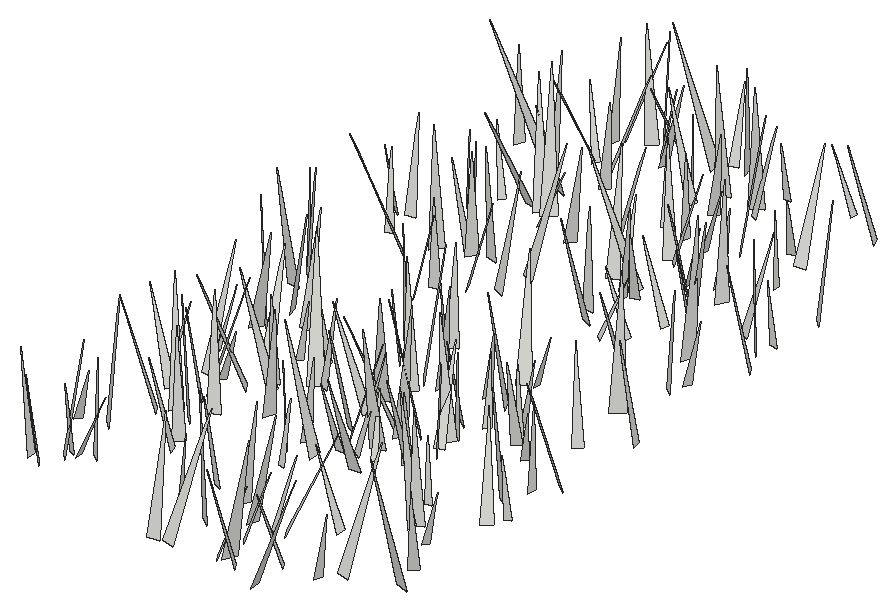
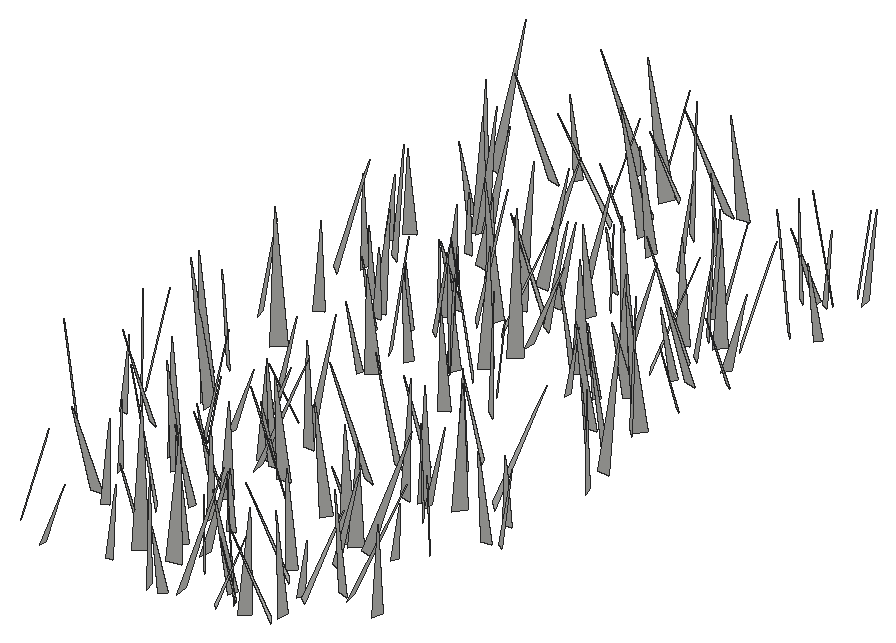
# SketchUp Ruby script. Lengths in inches.
U = 1.inch
M = Sketchup.active_model
def pt(a) = Geom::Point3d.new(a.map { |v| v * U })
def face(e, loops, mat)
  f = e.add_face(loops[0].map { |a| pt(a) })
  loops[1..].each { |l| e.add_face(l.map { |a| pt(a) }).erase! }
  f.material = f.back_material = mat if mat
  f
end
# faces: each face lists its corners as indices into pts; further lists are holes
def faces(e, pts, list, mat = nil) = list.each { |f| face(e, (f[0].is_a?(Array) ? f : [f]).map { |l| l.map { |i| pts[i] } }, mat) }
# xy, xz, yz: faces in a plane at the given z, y or x. An outline is a flat list of corners, or four numbers for a rectangle; further outlines are holes
def ring(l) = l.size == 4 ? [[l[0], l[1]], [l[2], l[1]], [l[2], l[3]], [l[0], l[3]]] : l.each_slice(2).to_a
def flat(e, list, mat, &to3) = list.each { |f| face(e, (f[0].is_a?(Array) ? f : [f]).map { |l| ring(l).map { |u, v| to3.(u, v) } }, mat) }
def xy(e, z, list, mat = nil) = flat(e, list, mat) { |x, y| [x, y, z] }
def xz(e, y, list, mat = nil) = flat(e, list, mat) { |x, z| [x, y, z] }
def yz(e, x, list, mat = nil) = flat(e, list, mat) { |y, z| [x, y, z] }
def lines(e, pts, list) = list.each { |a, b| e.add_line(pt(pts[a]), pt(pts[b])) }
# prism: a flat outline (further loops are holes) pulled along v
def prism(e, loops, v, mat = nil)
  f = face(e, loops, mat); d = Geom::Vector3d.new(v.map { |x| x * U })
  f.pushpull(f.normal.samedirection?(d) ? d.length : -d.length)
end
def box(e, o, s, mat = nil) = prism(e, [[o, [o[0] + s[0], o[1], o[2]], [o[0] + s[0], o[1] + s[1], o[2]], [o[0], o[1] + s[1], o[2]]]], [0, 0, s[2]], mat)
def at(x, y, z, deg = 0) = Geom::Transformation.translation(pt([x, y, z])) * Geom::Transformation.rotation(ORIGIN, Z_AXIS, deg.degrees)
def axes(o, x, y, z) = Geom::Transformation.new([*x, 0, *y, 0, *z, 0, *pt(o).to_a, 1])
def part(name) = M.definitions.add(name)
# library, detail: a bought-in or finely detailed component or shape, given as its bounding box
def library(name, o, s) = part(name).tap { |d| box(d.entities, o, s) }
def detail(e, o, s) = box(e.add_group.entities, o, s)
def put(e, d, t, mat = nil) = e.add_instance(d, t).tap { |i| i.material = mat if mat }
def group(e, t, mat = nil) = e.add_group.tap { |g| g.transformation = t; g.material = mat if mat }.entities
root = M.entities
c1 = part("fur_instance\#9")
p = [[0.8125,0,1.79],[0.67,-0.02,1.48],[0,-0.11,0],[0,0.11,0]]
faces(c1.entities,p,[[0,1,2,3]])
put(root,c1,axes([454.9,228.46,-21.66],[-2.14945,-3.42966,1.0737],[-3.50191,2.27993,0.27214],[0.80747,0.75821,4.03839]))
put(root,c1,axes([455.0625,214.63,-21.66],[-4.85936,-1.80324,2.4582],[-1.94231,5.39639,0.11902],[2.34986,0.73149,5.18178]))
put(root,c1,axes([455.69,246.77,-21.66],[-4.75498,1.70819,1.94206],[1.76287,5.11453,-0.18234],[1.89256,-0.47231,5.04921]))
put(root,c1,axes([456.17,210.82,-21.66],[-0.95753,-7.17721,1.84222],[-7.39469,1.0444,0.22542],[0.47406,1.79439,7.23729]))
put(root,c1,axes([456.03,213.25,-21.66],[3.99026,4.07334,2.14881],[4.32029,-4.29562,0.12027],[-1.59518,-1.44473,5.70086]))
put(root,c1,axes([456.43,228.82,-21.66],[-1.35199,5.16754,1.66066],[5.39955,1.4549,-0.13134],[0.55327,-1.57128,5.33986]))
put(root,c1,axes([457.3,168.51,-21.66],[4.90342,0.51596,3.18153],[0.4361,-5.84514,0.27581],[-3.19346,-0.00597,4.92277]))
put(root,c1,axes([456.92,224.95,-21.66],[-1.17354,4.22506,1.16991],[4.38332,1.15287,0.2334],[0.0799,-1.19029,4.3788]))
put(root,c1,axes([459.98,245.51,-21.66],[-7.66892,-1.90839,0.15613],[-1.91216,7.66661,-0.21311],[0.09999,0.24454,7.89993]))
put(root,c1,axes([456.22,177.14,-21.66],[3.1539,-2.32332,0.00557],[-2.32207,-3.15188,0.13648],[0.07647,0.11319,3.91488]))
put(root,c1,axes([459.46,187.51,-21.66],[-4.99004,2.24313,0.58277],[2.2784,5.00139,0.2583],[0.42444,-0.4756,5.46492]))
put(root,c1,axes([457.4375,189.73,-21.66],[2.29816,3.3477,0.63042],[3.39972,-2.30202,-0.16916],[-0.21536,-0.61617,4.05709]))
put(root,c1,axes([458.8125,167.71,-21.66],[3.31439,2.62679,2.62231],[3.03004,-3.94532,0.12232],[-2.14367,-1.5153,4.22732]))
put(root,c1,axes([460.44,222.64,-21.66],[-5.16383,-5.19186,0.43743],[-5.2089,5.15828,-0.26709],[0.11856,0.49863,7.31773]))
put(root,c1,axes([458.3,196.53,-21.66],[2.21445,2.95218,0.72503],[3.03203,-2.20951,-0.26401],[-0.21871,-0.73996,3.68096]))
put(root,c1,axes([459.07,202.87,-21.66],[-4.9247,-5.05159,2.9073],[-5.39927,5.38751,0.21521],[2.19519,1.91829,7.05159]))
put(root,c1,axes([459.38,233.9,-21.66],[3.09242,2.58599,1.68004],[2.84079,-3.31463,-0.12697],[-1.19992,-1.18273,4.02918]))
put(root,c1,axes([459.37,177.89,-21.66],[4.78863,4.89843,2.46119],[5.13986,-5.14824,0.24599],[-1.90629,-1.57608,6.84581]))
put(root,c1,axes([461.24,183.1,-21.66],[-5.49942,-3.45806,0.94275],[-3.51329,5.5426,-0.16378],[0.70973,0.64178,6.49422]))
put(root,c1,axes([459.34,206.71,-21.66],[5.12051,1.66894,1.66295],[1.70709,-5.37015,0.13306],[-1.62376,-0.38277,5.38398]))
put(root,c1,axes([460.07,171.33,-21.66],[-1.89592,-3.45095,1.30694],[-3.60556,2.04518,0.16982],[0.78554,1.05823,3.9338]))
put(root,c1,axes([461.32,236.99,-21.66],[-3.55756,1.9012,0.49829],[1.88183,3.59228,-0.2708],[0.56709,0.00632,4.02461]))
put(root,c1,axes([458.44,202.23,-21.66],[5.57249,-4.36069,0.56036],[-4.38496,-5.5781,0.19774],[-0.31889,0.50141,7.07313]))
put(root,c1,axes([459.89,170.41,-21.66],[-4.21577,-3.58718,3.5566],[-4.31781,4.96325,-0.11214],[2.62178,2.40587,5.53425]))
put(root,c1,axes([460.59,191.79,-21.66],[0.90222,6.95991,0.72818],[6.98982,-0.93156,0.24337],[-0.33621,-0.69025,7.01392]))
put(root,c1,axes([460.99,245.52,-21.66],[1.59622,5.71911,2.00108],[6.0184,-1.73595,0.16062],[-0.70101,-1.88115,5.93551]))
put(root,c1,axes([462.76,184.31,-21.66],[-5.4488,4.52209,1.619],[4.59694,5.6194,-0.22458],[1.39234,-0.85616,7.07731]))
put(root,c1,axes([463.16,248.99,-21.66],[-3.18461,-4.17271,0.10236],[-4.17132,3.18622,0.10881],[0.1486,0.01532,5.24799]))
put(root,c1,axes([462.46,225.35,-21.66],[-4.98307,4.13485,3.06586],[4.6284,5.46651,0.15019],[2.25263,-2.08511,6.47344]))
put(root,c1,axes([460.98,171.3,-21.66],[4.07736,0.20577,0.16386],[0.20057,-4.0788,0.13116],[-0.17019,0.12285,4.08044]))
put(root,c1,axes([462.42,172.05,-21.66],[-3.23296,-4.09809,2.47034],[-4.47809,3.64184,0.18098],[1.68632,1.81429,5.21667]))
put(root,c1,axes([462.55,204.81,-21.66],[-0.45657,6.34549,1.8425],[6.59681,0.54314,-0.23589],[0.37708,-1.81886,6.35752]))
put(root,c1,axes([463.32,187.54,-21.66],[-2.97615,-4.05495,1.48787],[-4.26463,3.04523,-0.23114],[0.68511,1.34083,5.02461]))
put(root,c1,axes([463.92,248.43,-21.66],[-3.60805,2.068,0.36238],[2.05277,3.62596,-0.25393],[0.44056,0.04128,4.15092]))
put(root,c1,axes([463.53,197.53,-21.66],[-2.14385,5.53708,0.23418],[5.53457,2.15208,-0.21752],[0.2875,-0.13964,5.93364]))
put(root,c1,axes([462.8,252.65,-21.66],[5.47635,-0.94494,2.24683],[-1.1073,-5.8869,0.22307],[-2.17142,0.61884,5.55279]))
put(root,c1,axes([465.27,192.08,-21.66],[-5.5722,-4.07145,0.43281],[-4.071,5.58734,0.1482],[0.43699,0.13539,6.89957]))
put(root,c1,axes([464.23,237.8,-21.66],[-1.51656,-6.50321,0.08888],[-6.50028,1.51258,-0.24097],[-0.21452,0.14123,6.67335]))
put(root,c1,axes([462.39,192.07,-21.66],[3.14021,-1.95272,0.11029],[-1.95573,-3.13292,0.21476],[0.01996,0.24059,3.6916]))
put(root,c1,axes([464.22,228.91,-21.66],[4.38059,2.58911,2.20412],[2.75267,-4.81057,0.18002],[-1.99611,-0.9519,5.08534]))
put(root,c1,axes([465.38,226.67,-21.66],[-4.97388,0.03891,0.99351],[0.0174,5.07103,-0.11152],[0.99411,0.10595,4.97278]))
put(root,c1,axes([464.99,241.65,-21.66],[-2.33347,-4.94017,0.88075],[-4.99474,2.38012,0.11709],[0.48332,0.74554,5.4623]))
put(root,c1,axes([465.86,237.4,-21.66],[-5.00326,5.02156,1.24961],[5.08502,5.09325,-0.10752],[0.95924,-0.80806,7.08781]))
put(root,c1,axes([463.3,253.92,-21.66],[4.56753,3.50086,0.36537],[3.49009,-4.58212,0.27435],[-0.45689,-0.00383,5.74831]))
put(root,c1,axes([464.92,183.58,-21.66],[4.55418,4.59674,3.34406],[5.23121,-5.06575,-0.16086],[-2.22422,-2.50228,6.46875]))
put(root,c1,axes([462.98,189.18,-21.66],[6.72571,2.73267,0.89443],[2.78268,-6.75899,-0.27437],[-0.72399,-0.59256,7.25447]))
put(root,c1,axes([465.95,254.65,-21.66],[-4.07853,4.6775,2.02917],[4.97181,4.22458,0.25488],[1.13033,-1.70436,6.20068]))
put(root,c1,axes([466.05,186.06,-21.66],[-2.20554,5.93145,2.00046],[6.2413,2.24627,0.22087],[0.47966,-1.95462,6.32437]))
put(root,c1,axes([466.94,237.33,-21.66],[-4.81371,6.17541,1.55135],[6.27572,4.93015,-0.15223],[1.07597,-1.1279,7.82843]))
put(root,c1,axes([467.84,193.06,-21.66],[-6.68615,-0.01766,0.93467],[0.01232,6.74773,0.2156],[0.93476,-0.21523,6.6827]))
put(root,c1,axes([467.42,177.96,-21.66],[-4.87581,-1.54153,0.97742],[-1.54685,4.96967,0.12147],[0.96896,0.17664,5.11224]))
put(root,c1,axes([466.73,179.75,-21.66],[3.45962,-4.50001,2.91683],[-5.02174,-3.93643,-0.1168],[-1.88153,2.2319,5.67498]))
put(root,c1,axes([466.07,226.34,-21.66],[4.61817,-3.87726,2.02523],[-4.05143,-4.90172,-0.14567],[-1.64942,1.18414,6.02822]))
put(root,c1,axes([465.95,199.66,-21.66],[3.13443,-2.25979,0.73802],[-2.32723,-3.16608,0.18952],[-0.4851,0.5876,3.85946]))
put(root,c1,axes([466.78,194.61,-21.66],[0.54293,-5.17192,1.62827],[-5.42158,-0.49338,0.24063],[0.08095,1.64396,5.19477]))
put(root,c1,axes([467.23,219.08,-21.66],[1.77747,-4.94769,1.74658],[-5.22789,-1.82695,0.145],[-0.44649,1.69476,5.25529]))
put(root,c1,axes([466.8,216.44,-21.66],[4.26525,2.34746,1.0733],[2.44325,-4.34035,-0.2164],[-0.83252,-0.71113,4.86375]))
put(root,c1,axes([468.62,200.81,-21.66],[-3.8802,0.07929,1.10053],[0.11582,4.03064,0.11798],[1.09728,-0.14508,3.87922]))
put(root,c1,axes([468.05,226.9375,-21.66],[-1.72933,-6.01967,2.37326],[-6.41752,1.90965,0.16749],[0.82719,2.23073,6.26091]))
put(root,c1,axes([469.16,255.27,-21.66],[-2.85386,-2.94003,0.13695],[-2.93623,2.85714,0.14971],[0.2028,-0.00613,4.09462]))
put(root,c1,axes([466.87,246.64,-21.66],[4.58247,4.01128,0.43645],[4.00699,-4.60163,0.22113],[-0.47421,-0.12046,6.08609]))
put(root,c1,axes([467.89,244.92,-21.66],[3.7544,-3.60472,1.46029],[-3.77286,-3.86843,0.15082],[-0.94444,1.12393,5.20257]))
put(root,c1,axes([468.47,253.24,-21.66],[-4.89725,-3.9807,3.26033],[-4.56553,5.43754,-0.21877],[2.37312,2.24631,6.30723]))
put(root,c1,axes([468.35,253.04,-21.66],[2.84043,2.51238,0.82611],[2.52394,-2.93724,0.2547],[-0.79009,-0.35083,3.78354]))
put(root,c1,axes([467.46,235.21,-21.66],[3.69637,0.13401,0.11411],[0.12786,-3.69317,0.19555],[-0.12096,0.19138,3.69362]))
put(root,c1,axes([470.29,196.71,-21.66],[-5.1988,6.07272,1.14347],[6.1224,5.26442,-0.12263],[0.83765,-0.78798,7.99315]))
put(root,c1,axes([469.53,252.04,-21.66],[5.0608,-1.8582,0.79428],[-1.91101,-5.09708,0.2516],[-0.65714,0.51221,5.38529]))
put(root,c1,axes([469.76,221.03,-21.66],[4.69401,2.26049,0.88712],[2.32694,-4.7392,-0.23643],[-0.69438,-0.60059,5.20458]))
put(root,c1,axes([470.56,189.1,-21.66],[5.91489,-2.56905,1.81184],[-2.61095,-6.16477,-0.21752],[-1.75092,0.51416,6.44505]))
put(root,c1,axes([473.71,254.89,-21.66],[-7.9003,-1.05971,0.99848],[-1.05239,7.96314,0.1246],[1.0062,0.00826,7.97008]))
put(root,c1,axes([471.23,196.77,-21.66],[1.95636,4.4496,1.57567],[4.70552,-1.97342,-0.26957],[-0.3738,-1.55425,4.8532]))
put(root,c1,axes([472.03,208.65,-21.66],[3.78368,4.97369,3.03573],[5.56614,-4.15585,-0.12867],[-1.72376,-2.50217,6.24798]))
put(root,c1,axes([471.875,234.46,-21.66],[4.94298,-3.20176,1.42299],[-3.34359,-5.04595,0.26096],[-1.0472,0.99819,5.88356]))
put(root,c1,axes([472.625,222.36,-21.66],[2.70818,5.99392,1.73773],[6.22026,-2.74585,-0.22279],[-0.5051,-1.67756,6.57356]))
put(root,c1,axes([473.96,205.26,-21.66],[-3.08736,-2.6391,1.38175],[-2.74426,3.29386,0.15946],[1.15895,0.7691,4.05847]))
put(root,c1,axes([473.11,226.25,-21.66],[2.96798,6.81466,1.03357],[6.887,-2.97737,-0.1458],[-0.27767,-1.00619,7.4315]))
put(root,c1,axes([476.4375,247.66,-21.66],[-5.80582,1.67481,0.45332],[1.66732,5.82342,-0.1609],[0.48013,0.02943,6.04042]))
put(root,c1,axes([474.4375,250.36,-21.66],[2.87799,2.64757,1.74089],[2.94858,-3.09885,-0.16173],[-1.16026,-1.30792,3.90721]))
put(root,c1,axes([474.9,256.24,-21.66],[-1.60634,4.05647,0.77587],[4.09581,1.67158,-0.25963],[0.53033,-0.623,4.35521]))
put(root,c1,axes([475.3,175.07,-21.66],[-2.10468,-4.52268,1.53831],[-4.75533,2.14388,-0.20306],[0.45584,1.48319,4.98428]))
put(root,c1,axes([474.8,169.88,-21.66],[4.07501,0.67414,1.38281],[0.80205,-4.27202,-0.28088],[-1.31276,-0.5174,4.12083]))
put(root,c1,axes([477.6875,195.53,-21.66],[-5.92651,0.06077,0.05927],[0.05827,5.92175,-0.24529],[0.06173,0.24468,5.92174]))
put(root,c1,axes([475.96,185.01,-21.66],[3.3067,2.95122,2.18217],[3.23124,-3.73382,0.15332],[-1.74087,-1.32466,4.4295]))
put(root,c1,axes([476.07,210.78,-21.66],[-2.39493,4.93051,2.15105],[5.27679,2.61079,-0.10925],[1.04521,-1.88321,5.4803]))
put(root,c1,axes([476.94,162.99,-21.66],[-0.4945,6.57851,1.5324],[6.75453,0.47319,0.14829],[-0.03697,-1.53911,6.5954]))
put(root,c1,axes([477.3,242.58,-21.66],[-1.55614,3.71904,0.91385],[3.82438,1.56093,0.15988],[0.20123,-0.90564,4.0283]))
put(root,c1,axes([476.7,256.12,-21.66],[5.38301,1.51294,2.42188],[1.75431,-5.82988,-0.25732],[-2.2532,-0.92457,5.58566]))
put(root,c1,axes([476.6,187.34,-21.66],[4.38951,-2.01268,1.547],[-2.15257,-4.58905,0.13732],[-1.34555,0.7756,4.82698]))
put(root,c1,axes([479.05,185.58,-21.66],[-7.32255,-0.11088,1.35528],[-0.08815,7.44603,0.13288],[1.35695,-0.11461,7.32218]))
put(root,c1,axes([477.77,250.9375,-21.66],[1.68119,-6.78383,2.85706],[-7.30642,-1.89388,-0.19753],[-0.89411,2.72073,6.98625]))
put(root,c1,axes([478.23,201.64,-21.66],[-4.52139,5.22079,2.42729],[5.56937,4.74843,0.161],[1.45961,-1.94607,6.90462]))
put(root,c1,axes([478.39,191.99,-21.66],[-3.05463,-4.97038,1.37571],[-5.09206,3.16016,0.11108],[0.81742,1.11209,5.83293]))
put(root,c1,axes([477.7,181.99,-21.66],[1.06055,3.50039,1.15885],[3.68372,-1.05849,-0.17402],[-0.16095,-1.16074,3.65339]))
put(root,c1,axes([477.28,198.17,-21.66],[4.02071,-6.30995,0.86141],[-6.36147,-4.02715,0.19326],[-0.29869,0.83076,7.47959]))
put(root,c1,axes([477.64,233.77,-21.66],[4.5925,4.65986,1.11021],[4.70947,-4.6734,0.13435],[-0.87619,-0.69491,6.5412]))
put(root,c1,axes([478.83,168.7,-21.66],[-4.49865,-5.44108,2.87885],[-5.83326,4.90701,0.15896],[1.96626,2.10876,7.05818]))
put(root,c1,axes([477.97,203.95,-21.66],[5.88152,4.86813,2.28116],[5.13014,-6.09312,-0.22398],[-1.60749,-1.63397,7.63157]))
put(root,c1,axes([479.67,231.42,-21.66],[-1.61925,6.67608,1.38838],[6.8184,1.60284,0.24489],[0.08425,-1.4073,6.86528]))
put(root,c1,axes([481.44,195.06,-21.66],[-5.39414,-3.77764,0.22745],[-3.78403,5.38986,-0.22257],[0.05845,0.31282,6.58162]))
put(root,c1,axes([478.67,163.12,-21.66],[1.55056,7.17303,0.47228],[7.18686,-1.53634,-0.26142],[0.15632,-0.51668,7.33405]))
put(root,c1,axes([480.32,187.94,-21.66],[-0.08561,-4.51883,0.61864],[-4.55746,0.06047,-0.18896],[-0.17898,0.62161,4.51569]))
put(root,c1,axes([483.22,230.95,-21.66],[-7.85705,-0.88135,0.16267],[-0.88597,7.85465,-0.23661],[0.1352,0.25331,7.90278]))
put(root,c1,axes([479.63,174.03,-21.66],[5.47744,-1.647,1.93505],[-1.81976,-5.75174,0.25556],[-1.77356,0.81501,5.71398]))
put(root,c1,axes([479.39,247.52,-21.66],[3.84963,-3.94903,0.87916],[-4.01863,-3.87266,0.20133],[-0.4673,0.77142,5.51126]))
put(root,c1,axes([480.64,204.47,-21.66],[-3.25997,-4.21096,1.97124],[-4.4396,3.53441,0.20814],[1.38129,1.42168,5.3213]))
put(root,c1,axes([480.38,241.84,-21.66],[4.66089,-0.94094,1.87831],[-0.93791,-5.02216,-0.1885],[-1.87983,0.17273,4.75118]))
put(root,c1,axes([481.64,237.8,-21.66],[-3.36286,5.21282,1.50099],[5.38655,3.41774,0.19865],[0.64152,-1.37145,6.20023]))
put(root,c1,axes([479.4375,190.77,-21.66],[5.1332,2.66859,0.80867],[2.72409,-5.16107,-0.26035],[-0.59552,-0.60587,5.77956]))
put(root,c1,axes([480.22,203.97,-21.66],[5.9168,-1.45412,1.7202],[-1.44139,-6.15974,-0.24915],[-1.73089,0.15879,6.08776]))
put(root,c1,axes([482.07,230.03,-21.66],[-0.89857,4.82904,0.37817],[4.8418,0.88433,0.21213],[-0.14006,-0.41036,4.90735]))
put(root,c1,axes([481.63,225,-21.66],[0.33576,5.45677,2.6197],[6.05197,-0.25349,-0.24764],[0.11336,-2.62894,5.46148]))
put(root,c1,axes([481.9375,250.99,-21.66],[3.60415,-6.43604,2.10161],[-6.7075,-3.71823,0.11619],[-0.92131,1.89247,7.37557]))
put(root,c1,axes([483.01,223.08,-21.66],[-2.27159,-6.08211,1.19958],[-6.16809,2.34544,0.21162],[0.62109,1.04786,6.48903]))
put(root,c1,axes([482,188.47,-21.66],[3.27247,4.57721,0.86039],[4.6176,-3.3258,0.13012],[-0.60735,-0.62316,5.62521]))
put(root,c1,axes([484.55,195.26,-21.66],[-5.73221,-5.07274,1.73381],[-5.23258,5.8463,-0.19467],[1.1657,1.29813,7.652]))
put(root,c1,axes([482.97,190.55,-21.66],[2.46891,-7.20313,1.70316],[-7.36136,-2.57683,-0.22704],[-0.77207,1.53499,7.61111]))
put(root,c1,axes([482.83,249.52,-21.66],[2.64907,4.14771,0.84835],[4.17625,-2.72433,0.27885],[-0.69438,-0.56151,4.91358]))
put(root,c1,axes([482.47,237.32,-21.66],[3.7464,3.46532,0.67043],[3.46985,-3.79505,0.22613],[-0.64655,-0.28736,5.09832]))
put(root,c1,axes([483.2,254.29,-21.66],[0.28978,-3.77503,0.68612],[-3.83038,-0.24462,0.27184],[0.22308,0.70349,3.77636]))
put(root,c1,axes([482.98,228.84,-21.66],[5.23095,-0.44242,1.6949],[-0.413,-5.49862,-0.16069],[-1.70231,-0.02548,5.24716]))
put(root,c1,axes([484.17,188.49,-21.66],[-1.12302,3.48075,0.37457],[3.50037,1.10997,0.18007],[-0.0574,-0.41163,3.65299]))
put(root,c1,axes([483.9,185.78,-21.66],[0.0355,-6.28923,0.69696],[-6.32457,-0.05728,-0.19472],[-0.19984,0.69551,6.28631]))
put(root,c1,axes([483.15,193.83,-21.66],[6.93717,-2.75986,2.51351],[-2.97128,-7.29338,0.19237],[-2.25967,1.11744,7.46352]))
put(root,c1,axes([482.59,171.47,-21.66],[6.6153,-1.38256,1.33275],[-1.44359,-6.733,0.18083],[-1.26639,0.45296,6.75581]))
put(root,c1,axes([483.39,241.04,-21.66],[4.21997,-0.6182,0.41958],[-0.60999,-4.24047,-0.11271],[-0.43142,-0.05127,4.26352]))
put(root,c1,axes([483.88,229.58,-21.66],[1.95757,-4.55386,0.31612],[-4.56359,-1.94437,0.25034],[0.10577,0.38911,4.95045]))
put(root,c1,axes([484.25,168.05,-21.66],[3.13129,2.44329,0.37399],[2.42945,-3.15346,0.26073],[-0.45532,-0.0231,3.96316]))
put(root,c1,axes([486.15,209.33,-21.66],[-3.98192,5.65644,1.02142],[5.69703,4.04883,-0.21229],[0.76316,-0.7113,6.91418]))
put(root,c1,axes([484.28,163.78,-21.66],[3.52648,2.43175,0.31475],[2.41999,-3.54045,0.23962],[-0.3951,0.0194,4.27692]))
put(root,c1,axes([485.2,171.4,-21.66],[2.13777,3.57515,0.4757],[3.58502,-2.16686,0.17428],[-0.39447,-0.3179,4.1619]))
put(root,c1,axes([486.72,163.58,-21.66],[-4.48858,-3.56813,1.07524],[-3.58767,4.5928,0.2643],[1.00813,0.45789,5.72792]))
put(root,c1,axes([486.35,199.55,-21.66],[-2.7828,-3.97435,1.2381],[-4.07565,2.90431,0.16237],[0.84701,0.91751,4.84903]))
put(root,c1,axes([484.92,205.32,-21.66],[3.8804,-2.67072,0.47699],[-2.66948,-3.90717,-0.15997],[-0.48385,0.13783,4.70793]))
put(root,c1,axes([487.54,196.04,-21.66],[-5.4066,3.91291,1.98693],[4.14231,5.59139,0.26032],[1.44915,-1.38406,6.66892]))
put(root,c1,axes([487.4,205.02,-21.66],[-5.57513,-2.9786,1.92177],[-3.03694,5.86084,0.2736],[1.82819,0.65252,6.315]))
put(root,c1,axes([485.19,164.64,-21.66],[6.75458,-3.1446,1.55563],[-3.25939,-6.87331,0.25842],[-1.29802,0.89549,7.44621]))
put(root,c1,axes([488.34,222.86,-21.66],[-3.79909,0.62191,0.11225],[0.62576,3.79759,0.13861],[0.08831,-0.15497,3.84716]))
put(root,c1,axes([487.61,194.37,-21.66],[-1.13883,5.42731,0.08742],[5.42427,1.13458,0.2244],[-0.2017,-0.13157,5.54096]))
put(root,c1,axes([486.03,221.3,-21.66],[2.19151,2.85606,0.09461],[2.85445,-2.18225,-0.24214],[0.13471,-0.22234,3.59182]))
put(root,c1,axes([486.34,234.68,-21.66],[3.55375,0.65284,0.74182],[0.70307,-3.6162,-0.18565],[-0.69441,-0.32026,3.60844]))
put(root,c1,axes([486.06,243.33,-21.66],[6.38411,4.40631,2.11358],[4.61615,-6.57865,-0.22824],[-1.60436,-1.39477,7.75373]))
put(root,c1,axes([487.67,197.04,-21.66],[2.36348,3.65871,1.87372],[3.9267,-2.64879,0.21906],[-1.21573,-1.4425,4.3502]))
put(root,c1,axes([487.22,189.82,-21.66],[2.10827,-4.41232,0.88185],[-4.4927,-2.11805,0.1432],[-0.24874,0.85808,4.88803]))
put(root,c1,axes([489.6875,226.97,-21.66],[-4.67921,0.76999,0.1435],[0.76372,4.67821,-0.1991],[0.17382,0.17327,4.73796]))
put(root,c1,axes([487.26,210.06,-21.66],[3.61055,-0.61097,0.20103],[-0.59508,-3.6081,-0.27795],[-0.24409,-0.24103,3.65131]))
put(root,c1,axes([488.25,193.12,-21.66],[-3.74017,-2.83655,2.38458],[-3.12746,4.23356,0.13062],[1.98777,1.32365,4.69232]))
put(root,c1,axes([488.75,200.5,-21.66],[-3.06481,2.41196,1.362],[2.48233,3.29293,-0.24563],[1.22908,-0.63618,3.89234]))
put(root,c1,axes([486.43,171.79,-21.66],[5.74165,3.30721,0.02247],[3.30582,-5.73764,-0.2359],[0.09829,-0.21562,6.62182]))
put(root,c1,axes([490.47,175.39,-21.66],[-4.67838,0.58429,0.4377],[0.60816,4.68963,0.24018],[0.40387,-0.29353,4.7086]))
put(root,c1,axes([490.24,255.84,-21.66],[-3.8674,0.14725,0.40736],[0.1724,3.88071,0.23399],[0.39736,-0.25058,3.86312]))
put(root,c1,axes([490.3125,166.56,-21.66],[-3.61255,-2.36918,0.54232],[-2.35627,3.65218,0.25916],[0.59592,0.07847,4.31235]))
put(root,c1,axes([490.73,230.05,-21.66],[3.77255,3.78798,3.73229],[4.48771,-4.72284,0.25719],[-2.85294,-2.4201,5.33992]))
put(root,c1,axes([490.39,229.82,-21.66],[-3.18222,-1.83698,0.96818],[-1.93012,3.2701,-0.13938],[0.76583,0.60852,3.67173]))
put(root,c1,axes([490.24,219.15,-21.66],[-1.40933,-4.17013,0.64925],[-4.20295,1.44894,0.18319],[0.38311,0.55526,4.39803]))
put(root,c1,axes([489.01,236.44,-21.66],[4.9839,-2.53795,0.76874],[-2.53211,-5.04073,-0.2255],[-0.78777,0.14572,5.58834]))
put(root,c1,axes([491.09,186.24,-21.66],[-1.0754,-7.3325,1.08617],[-7.40599,1.10888,0.15329],[0.31086,1.05196,7.40935]))
put(root,c1,axes([491,234.25,-21.66],[-5.47966,3.19166,2.7493],[3.39794,6.01513,-0.2105],[2.48986,-1.18473,6.33791]))
put(root,c1,axes([490.26,246.02,-21.66],[1.67975,-3.93598,0.16611],[-3.93538,-1.66827,0.26597],[0.17974,0.25696,4.27115]))
put(root,c1,axes([491.41,202.77,-21.66],[3.83893,-0.81047,1.08867],[-0.8917,-3.9684,0.19003],[-1.0232,0.41758,3.91895]))
put(root,c1,axes([492.52,244.56,-21.66],[-0.48607,6.36101,0.33267],[6.36907,0.48063,0.1158],[-0.09028,-0.34048,6.37851]))
put(root,c1,axes([492.76,200.5,-21.66],[-0.42877,3.87256,1.55947],[4.17346,0.35848,0.25729],[-0.1042,-1.57711,3.88772]))
put(root,c1,axes([490.62,161.79,-21.66],[6.76067,1.19839,0.69108],[1.18973,-6.79585,0.14582],[-0.7059,0.02372,6.86451]))
put(root,c1,axes([493.28,239.91,-21.66],[-3.94466,-0.14605,1.57067],[-0.23954,4.23653,-0.20765],[1.55915,0.28136,3.94189]))
put(root,c1,axes([493.13,199.6,-21.66],[2.16413,-4.87719,1.14426],[-4.95965,-2.26151,-0.2591],[-0.70577,0.93721,5.32947]))
put(root,c1,axes([493.76,184.93,-21.66],[-0.42673,3.51272,1.26133],[3.73148,0.37463,0.21911],[-0.0791,-1.27778,3.53176]))
put(root,c1,axes([495.14,253.01,-21.66],[-4.90258,-2.23132,0.87524],[-2.28191,4.95484,-0.15015],[0.73329,0.50088,5.38438]))
put(root,c1,axes([495.38,180.78,-21.66],[-7.11208,1.53537,2.26223],[1.65379,7.4363,0.15223],[2.17716,-0.6331,7.27433]))
put(root,c1,axes([495.52,181.02,-21.66],[3.10657,-5.20372,2.6425],[-5.63717,-3.45056,-0.16782],[-1.51121,2.17421,6.05816]))
put(root,c1,axes([494.48,166.84,-21.66],[4.0424,-1.6774,0.68877],[-1.67315,-4.09915,-0.16314],[-0.69903,0.11126,4.37357]))
put(root,c1,axes([494.57,224.4,-21.66],[7.78387,0.2727,2.09642],[0.3333,-8.05673,-0.18953],[-2.08764,-0.26953,7.78634]))
put(root,c1,axes([495.4,223.57,-21.66],[7.52534,-2.11015,2.94691],[-2.32099,-8.02168,0.183],[-2.78389,0.98374,7.81345]))
put(root,c1,axes([495.57,197.8125,-21.66],[2.79472,-2.37927,0.19168],[-2.37504,-2.80125,-0.14262],[-0.23842,0.01542,3.66757]))
put(root,c1,axes([496.72,210.88,-21.66],[4.92232,-5.34816,3.43981],[-5.97476,-5.37881,0.1869],[-2.17654,2.67018,7.26616]))
put(root,c1,axes([496.08,168.68,-21.66],[1.83288,7.01444,0.75411],[7.05484,-1.82448,-0.17632],[-0.01908,-0.77421,7.24781]))
put(root,c1,axes([498.02,202.96,-21.66],[2.13883,-4.28297,3.06723],[-5.00629,-2.68295,-0.2554],[-1.63976,2.60467,4.7805]))
put(root,c1,axes([496.72,230.58,-21.66],[2.68485,5.08236,0.90598],[5.15716,-2.6868,-0.21076],[-0.23424,-0.9002,5.74408]))
put(root,c1,axes([498.01,217.17,-21.66],[3.30572,4.13092,2.03155],[4.38871,-3.58299,0.14433],[-1.38957,-1.489,5.28881]))
put(root,c1,axes([498.94,190.05,-21.66],[3.12486,4.78234,3.10342],[5.39282,-3.6275,0.15986],[-1.8492,-2.49745,5.71052]))
put(root,c1,axes([498.44,178.65,-21.66],[3.31097,-1.72543,0.32906],[-1.73993,-3.31791,0.10944],[-0.24091,0.24944,3.73197]))
put(root,c1,axes([498.66,219.36,-21.66],[3.79566,-1.87078,0.73995],[-1.92959,-3.83243,0.2087],[-0.56925,0.51676,4.2265]))
put(root,c1,axes([500.67,185.4375,-21.66],[-3.10471,5.12305,0.88051],[5.18598,3.12286,0.11631],[0.35573,-0.81381,5.98927]))
put(root,c1,axes([499.75,228.6,-21.66],[4.37424,4.04681,2.79179],[4.54542,-4.75288,-0.23239],[-1.87347,-2.08284,5.95454]))
put(root,c1,axes([499.97,193.375,-21.66],[-4.58199,0.67037,2.42399],[0.81188,5.16228,0.10702],[2.38033,-0.47034,4.62953]))
put(root,c1,axes([500.37,230.625,-21.66],[0.0054,-4.02258,1.09842],[-4.16704,0.03516,0.14925],[0.15324,1.09787,4.01982]))
put(root,c1,axes([501.75,225.33,-21.66],[-4.7875,-3.33897,1.34753],[-3.4677,4.87923,-0.23006],[0.96934,0.96392,5.83232]))
put(root,c1,axes([501.96,195.48,-21.66],[-3.86878,-4.9807,0.99535],[-5.05831,3.89149,-0.18804],[0.45997,0.9025,6.30392]))
put(root,c1,axes([502.15,206.93,-21.66],[-5.31437,-1.63311,1.48269],[-1.72892,5.48589,-0.1545],[1.36976,0.58821,5.55749]))
put(root,c1,axes([500.86,236.99,-21.66],[4.54729,4.68314,2.12923],[4.88324,-4.82336,0.17985],[-1.61844,-1.39522,6.52513]))
put(root,c1,axes([501.67,187.49,-21.66],[0.6335,-3.36408,1.34348],[-3.58683,-0.77327,-0.24494],[-0.50657,1.2682,3.41444]))
put(root,c1,axes([500.69,174.02,-21.66],[3.52243,-4.25283,0.7835],[-4.27225,-3.57882,-0.21878],[-0.66956,0.46198,5.5178]))
put(root,c1,axes([502.04,170.46,-21.66],[-2.39726,-7.68863,1.50052],[-7.81274,2.46126,0.12966],[0.5725,1.39306,8.05265]))
